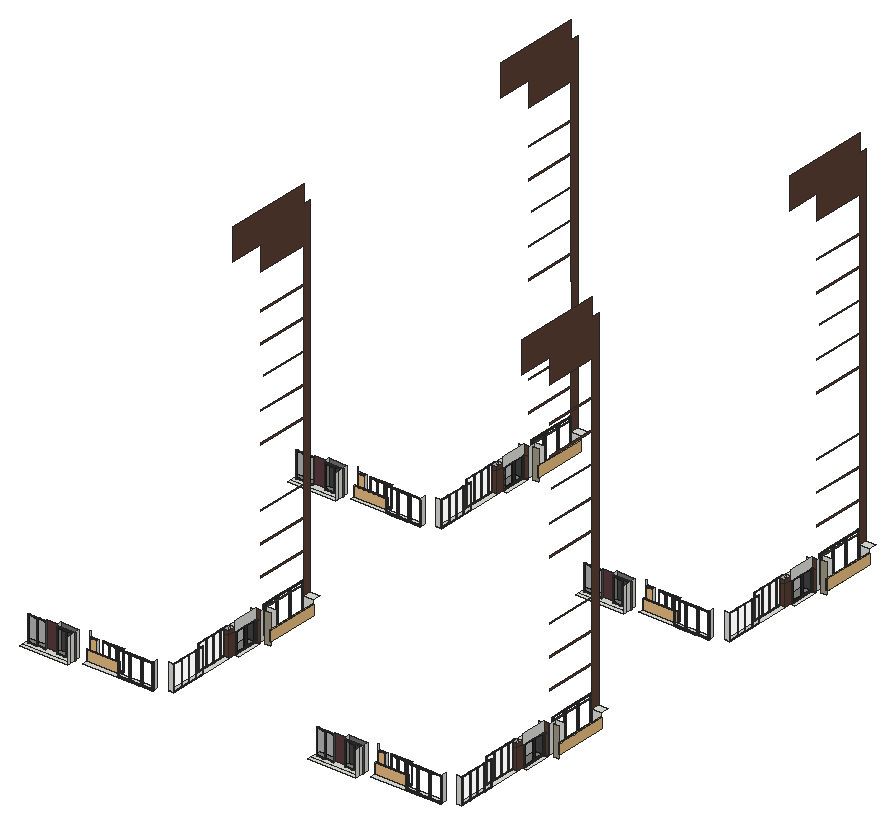
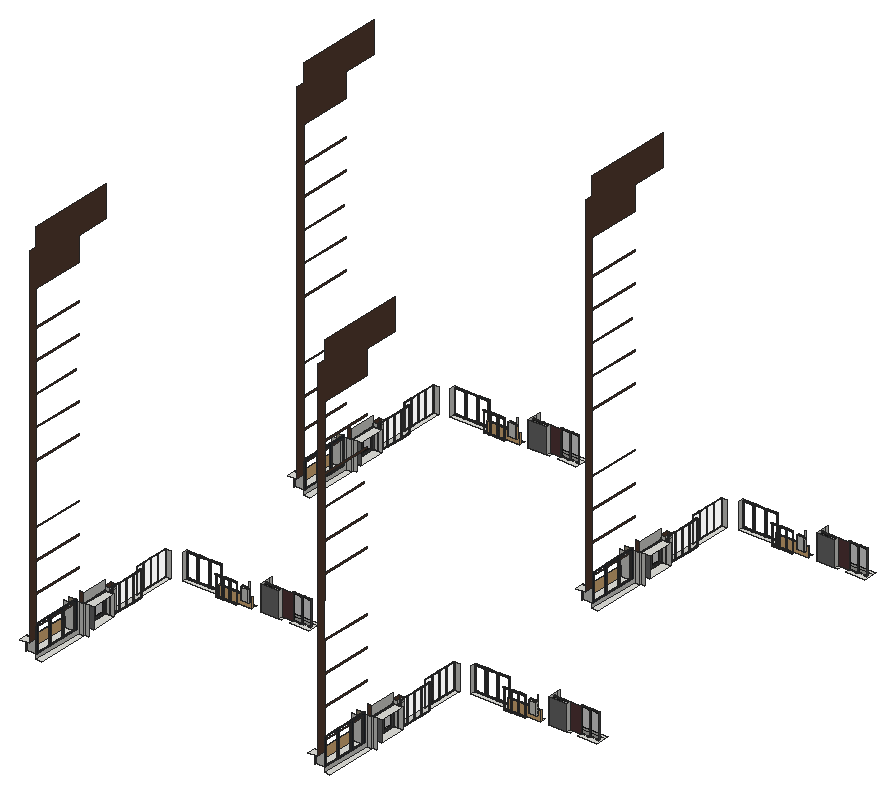
# SketchUp Ruby script. Lengths in inches.
U = 1.inch
M = Sketchup.active_model
def pt(a) = Geom::Point3d.new(a.map { |v| v * U })
def face(e, loops, mat)
  f = e.add_face(loops[0].map { |a| pt(a) })
  loops[1..].each { |l| e.add_face(l.map { |a| pt(a) }).erase! }
  f.material = f.back_material = mat if mat
  f
end
# faces: each face lists its corners as indices into pts; further lists are holes
def faces(e, pts, list, mat = nil) = list.each { |f| face(e, (f[0].is_a?(Array) ? f : [f]).map { |l| l.map { |i| pts[i] } }, mat) }
# xy, xz, yz: faces in a plane at the given z, y or x. An outline is a flat list of corners, or four numbers for a rectangle; further outlines are holes
def ring(l) = l.size == 4 ? [[l[0], l[1]], [l[2], l[1]], [l[2], l[3]], [l[0], l[3]]] : l.each_slice(2).to_a
def flat(e, list, mat, &to3) = list.each { |f| face(e, (f[0].is_a?(Array) ? f : [f]).map { |l| ring(l).map { |u, v| to3.(u, v) } }, mat) }
def xy(e, z, list, mat = nil) = flat(e, list, mat) { |x, y| [x, y, z] }
def xz(e, y, list, mat = nil) = flat(e, list, mat) { |x, z| [x, y, z] }
def yz(e, x, list, mat = nil) = flat(e, list, mat) { |y, z| [x, y, z] }
def lines(e, pts, list) = list.each { |a, b| e.add_line(pt(pts[a]), pt(pts[b])) }
# prism: a flat outline (further loops are holes) pulled along v
def prism(e, loops, v, mat = nil)
  f = face(e, loops, mat); d = Geom::Vector3d.new(v.map { |x| x * U })
  f.pushpull(f.normal.samedirection?(d) ? d.length : -d.length)
end
def box(e, o, s, mat = nil) = prism(e, [[o, [o[0] + s[0], o[1], o[2]], [o[0] + s[0], o[1] + s[1], o[2]], [o[0], o[1] + s[1], o[2]]]], [0, 0, s[2]], mat)
def at(x, y, z, deg = 0) = Geom::Transformation.translation(pt([x, y, z])) * Geom::Transformation.rotation(ORIGIN, Z_AXIS, deg.degrees)
def axes(o, x, y, z) = Geom::Transformation.new([*x, 0, *y, 0, *z, 0, *pt(o).to_a, 1])
def part(name) = M.definitions.add(name)
# library, detail: a bought-in or finely detailed component or shape, given as its bounding box
def library(name, o, s) = part(name).tap { |d| box(d.entities, o, s) }
def detail(e, o, s) = box(e.add_group.entities, o, s)
def put(e, d, t, mat = nil) = e.add_instance(d, t).tap { |i| i.material = mat if mat }
def group(e, t, mat = nil) = e.add_group.tap { |g| g.transformation = t; g.material = mat if mat }.entities
root = M.entities
M.materials.add("Glass_Tinted_Gray").color = [0, 0, 0]
M.materials["Glass_Tinted_Gray"].alpha = 0.125
M.materials.add("Glazing").color = [128, 128, 128]
M.materials["Glazing"].alpha = 0.05
M.materials.add("Powdercoating").color = [41, 44, 40]
M.materials.add("Wine2").color = [0, 0, 0]
M.materials["Wine2"].alpha = 0
M.materials.add("[0130_Gainsboro]").color = [39, 45, 50]
M.materials.add("[0135_DarkGray]").color = [81, 81, 81]
M.materials.add("[Color M05]").color = [114, 114, 114]
M.materials.add("[Concrete Tile]").color = [165, 155, 133]
M.materials.add("[Granite Brown]").color = [89, 59, 61]
M.materials.add("[Granite Brown]1").color = [89, 63, 50]
M.materials.add("[Mirror 02]").color = [229, 229, 229]
M.materials.add("[Terrazzo Light Blue]").color = [196, 214, 227]
c1 = part("PENTEK_RP Fineline 50S_Sliding_DoorCase_E1")
box(c1.entities,[0,0,0],[1.51,3.66,99.27],"[0135_DarkGray]")
c2 = part("PENTEK_RP Fineline 50S_SlidingDooe_Case_E2")
box(c2.entities,[0,0,0],[96.25,3.66,1.51],"[0135_DarkGray]")
c3 = part("pentek_RP Fineline 50S_SlidingDoor_Case")
put(c3.entities,c1,at(97.76,0,0))
put(c3.entities,c2,at(1.51,0,0))
put(c3.entities,c1,at(0,0,0))
put(c3.entities,c2,at(1.51,0,97.76))
c4 = part("PENTEK_RP Fineline 50S_SlidingDoor_GlazingBead_2")
box(c4.entities,[0,0,0],[0.56,0.59,94.39],"[0135_DarkGray]")
c5 = part("PENTEK_RP Fineline 50S_SlidingDoor_Glass")
box(c5.entities,[0,0,0],[46.58,0.16,94.39],"Glass_Tinted_Gray")
c6 = part("PENTEK_RP Fineline 50S_SlidingDoor_GlazingBead")
box(c6.entities,[0,0,0],[45.47,0.59,0.56],"[0135_DarkGray]")
c7 = part("PENTEK_RP Fineline 50S_SlidingDoor_Leaf_E1")
xy(c7.entities,0,[[0,0,0.93,1.97],[0.93,1.57,1.49,1.97]],"[0135_DarkGray]")
xy(c7.entities,96.25,[[0,0,0.93,0,0.93,1.57,1.49,1.57,1.49,1.97,0,1.97]],"[0135_DarkGray]")
xz(c7.entities,0,[[0,0,0.93,96.25]],"[0135_DarkGray]")
xz(c7.entities,1.57,[[0.93,0,1.49,95.32],[0.93,95.32,1.49,96.25]],"[0135_DarkGray]")
xz(c7.entities,1.97,[[0,0,1.49,96.25]],"[0135_DarkGray]")
yz(c7.entities,0,[[0,0,1.97,96.25]],"[0135_DarkGray]")
yz(c7.entities,0.93,[[0,0,1.57,0.93],[0,0.93,1.57,95.32],[0,95.32,1.57,96.25]],"[0135_DarkGray]")
yz(c7.entities,1.49,[[1.57,0,1.97,95.32],[1.57,95.32,1.97,96.25]],"[0135_DarkGray]")
c8 = part("PENTEK_RP Fineline 50S_SlidingDoor_Leaf_E2")
xy(c8.entities,0,[[0,0,0,1.57,0.56,1.57,0.56,1.97,46.02,1.97,46.02,1.57,46.58,1.57,46.58,0]],"[0135_DarkGray]")
xy(c8.entities,0.93,[[0,0,46.58,1.57]],"[0135_DarkGray]")
xy(c8.entities,1.49,[[0.56,1.57,46.02,1.97]],"[0135_DarkGray]")
xz(c8.entities,0,[[0,0,46.58,0.93]],"[0135_DarkGray]")
xz(c8.entities,1.57,[[0,0,0.56,0.93],[46.02,0,46.58,0.93],[0.56,0.93,46.02,1.49]],"[0135_DarkGray]")
xz(c8.entities,1.97,[[0.56,0,46.02,1.49]],"[0135_DarkGray]")
yz(c8.entities,0,[[0,0,1.57,0.93]],"[0135_DarkGray]")
yz(c8.entities,0.56,[[1.57,0,1.97,0.93],[1.57,0.93,1.97,1.49]],"[0135_DarkGray]")
yz(c8.entities,46.02,[[1.57,0,1.97,0.93],[1.57,0.93,1.97,1.49]],"[0135_DarkGray]")
yz(c8.entities,46.58,[[0,0,1.57,0.93]],"[0135_DarkGray]")
c9 = part("PENTEK_RP Fineline S_SlidingDoor_Leaf1")
put(c9.entities,c4,at(0.93,0,0.93))
put(c9.entities,c4,at(46.96,0,0.93))
put(c9.entities,c5,at(1.49,1.42,0.93))
put(c9.entities,c6,at(1.49,0,0.93))
put(c9.entities,c5,at(1.49,0.59,0.93),"[Terrazzo Light Blue]")
put(c9.entities,c7,at(0,0,0))
put(c9.entities,c7,axes([48.44,0,0],[-1,0,0],[0,1,0],[0,0,1]))
put(c9.entities,c8,axes([0.93,0,96.25],[1,0,0],[0,1,0],[0,0,-1]))
put(c9.entities,c8,at(0.93,0,0))
put(c9.entities,c6,at(1.49,0,94.77))
c10 = part("PENTEK_RP Fineline 50S_SlidingDoor_Leaf2")
put(c10.entities,c5,at(1.49,1.42,0.93))
put(c10.entities,c6,at(1.49,0,94.77))
put(c10.entities,c4,at(46.96,0,0.93))
put(c10.entities,c5,at(1.49,0.59,0.93),"[Mirror 02]")
put(c10.entities,c4,at(0.93,0,0.93))
put(c10.entities,c7,at(0,0,0))
put(c10.entities,c7,axes([48.44,0,0],[-1,0,0],[0,1,0],[0,0,1]))
put(c10.entities,c6,at(1.49,0,0.93))
put(c10.entities,c8,axes([0.93,0,96.25],[1,0,0],[0,1,0],[0,0,-1]))
put(c10.entities,c8,at(0.93,0,0))
c11 = part("PENTEK - Slimmest Steel Sliding Door / Window\#1")
put(c11.entities,c3,at(0,-1.88,-0.09))
put(c11.entities,c9,at(1.51,-2.27,1.42))
put(c11.entities,c10,at(49.32,-0.3,1.42))
c12 = part("Group\#15")
xy(c12.entities,0,[[0,-55.94,0.71,45.94]])
xy(c12.entities,0.2,[[0,-55.94,0.47,45.94],[0.47,45.94,0.71,46.42]])
xy(c12.entities,2.36,[[0.47,-55.94,0.71,46.42]])
xz(c12.entities,-55.94,[[0,0,0.71,0,0.71,2.36,0.47,2.36,0.47,0.2,0,0.2]])
xz(c12.entities,45.94,[[0,0,0.71,0.2]])
xz(c12.entities,46.42,[[0.47,0.2,0.71,2.36]])
yz(c12.entities,0,[[-55.94,0,45.94,0.2]])
yz(c12.entities,0.47,[[-55.94,0.2,46.42,2.36]])
yz(c12.entities,0.71,[[-55.94,0,45.94,0,45.94,0.2,46.42,0.2,46.42,2.36,-55.94,2.36]])
c13 = part("Group\#7")
xy(c13.entities,0,[[0,-59.09,0.71,45.94]])
xy(c13.entities,0.2,[[0,-59.09,0.47,45.94],[0.47,45.94,0.71,46.42]])
xy(c13.entities,2.36,[[0.47,-59.09,0.71,46.42]])
xz(c13.entities,-59.09,[[0,0,0.71,0,0.71,2.36,0.47,2.36,0.47,0.2,0,0.2]])
xz(c13.entities,45.94,[[0,0,0.71,0.2]])
xz(c13.entities,46.42,[[0.47,0.2,0.71,2.36]])
yz(c13.entities,0,[[-59.09,0,45.94,0.2]])
yz(c13.entities,0.47,[[-59.09,0.2,46.42,2.36]])
yz(c13.entities,0.71,[[-59.09,0,45.94,0,45.94,0.2,46.42,0.2,46.42,2.36,-59.09,2.36]])
c14 = part("Group\#16")
prism(c14.entities,[[[0.47,-56.18,0.2],[0,-56.18,0.2],[0,-56.18,0],[0.71,-56.18,0],[0.71,-56.18,2.36],[0.47,-56.18,2.36]]],[0,28.68,0])
c15 = part("Group\#10")
box(c15.entities,[-0.73,0,0],[27.99,0.55,102.05])
c16 = part("Group\#18")
xy(c16.entities,0,[[0.47,-56.18,0.47,-55.47,0,-55.47,0,-28.21,1.18,-28.21,1.18,-56.18]])
xy(c16.entities,0.2,[[0.71,-56.18,1.18,-28.21],[0,-55.47,0.47,-28.21],[0.47,-28.21,0.71,-27.74]])
xy(c16.entities,2.36,[[0.47,-56.18,0.71,-27.74]])
xz(c16.entities,-56.18,[[0.47,0,1.18,0,1.18,0.2,0.71,0.2,0.71,2.36,0.47,2.36]])
xz(c16.entities,-55.47,[[0,0,0.47,0.2]])
xz(c16.entities,-28.21,[[0,0,1.18,0.2]])
xz(c16.entities,-27.74,[[0.47,0.2,0.71,2.36]])
yz(c16.entities,0,[[-55.47,0,-28.21,0.2]])
yz(c16.entities,0.47,[[-56.18,0,-55.47,0.2],[-56.18,0.2,-27.74,2.36]])
yz(c16.entities,0.71,[[-56.18,0.2,-27.74,2.36]])
yz(c16.entities,1.18,[[-56.18,0,-28.21,0.2]])
c17 = part("Group\#34")
xy(c17.entities,0,[[-20.45,0,7.76,1.22]])
xy(c17.entities,0.06,[[-20.39,0.06,7.7,1.22]])
xy(c17.entities,0.47,[[-19.98,0,7.28,0.06]])
xy(c17.entities,101.89,[[-19.98,0,7.28,0.06]])
xy(c17.entities,102.3,[[-20.39,0.06,7.7,1.22]])
xy(c17.entities,102.36,[[-20.45,0,7.76,1.22]])
xz(c17.entities,0,[[[-20.45,0,7.76,102.36],[-19.98,0.47,7.28,101.89]]])
xz(c17.entities,0.06,[[[-20.39,0.06,7.7,102.3],[-19.98,0.47,7.28,101.89]]])
xz(c17.entities,1.22,[[[-20.45,0,7.76,102.36],[-20.39,0.06,7.7,102.3]]])
yz(c17.entities,-20.45,[[0,0,1.22,102.36]])
yz(c17.entities,-20.39,[[0.06,0.06,1.22,102.3]])
yz(c17.entities,-19.98,[[0,0.47,0.06,101.89]])
yz(c17.entities,7.28,[[0,0.47,0.06,101.89]])
yz(c17.entities,7.7,[[0.06,0.06,1.22,102.3]])
yz(c17.entities,7.76,[[0,0,1.22,102.36]])
c18 = part("Group\#6")
put(c18.entities,c12,axes([27.97,0,7.875],[1,0,0],[0,0,-1],[0,1,0]),"Powdercoating")
put(c18.entities,c13,axes([0.71,0,6.8],[-1,0,0],[0,0,-0.97687],[0,1,0]),"Powdercoating")
put(c18.entities,c14,axes([-27.5,0,-38.07],[0,0,-1],[-1,0,0],[0,1,0]),"Powdercoating")
put(c18.entities,c15,at(1.12,0.35,-38.39),"Glazing")
put(c18.entities,c16,axes([-27.5,0,63.35],[0,0,1],[-1,0,0],[0,1,0]),"Powdercoating")
put(c18.entities,c17,at(20.6875,1.0625,-38.54),"Powdercoating")
c19 = part("Sliding door assembly")
put(c19.entities,c18,at(-1.18,4.5,38.86))
g1 = group(c19.entities,at(84.74,4.5,38.86))
put(g1,c12,axes([-27.97,0,7.875],[-1,0,0],[0,0,-1],[0,1,0]),"Powdercoating")
put(g1,c13,axes([-0.71,0,6.8],[1,0,0],[0,0,-0.97687],[0,1,0]),"Powdercoating")
put(g1,c14,axes([27.5,0,-38.07],[0,0,-1],[1,0,0],[0,1,0]),"Powdercoating")
put(g1,c15,axes([-1.12,0.35,-38.39],[-1,0,0],[0,1,0],[0,0,1]),"Glazing")
put(g1,c16,axes([27.5,0,63.35],[0,0,1],[1,0,0],[0,1,0]),"Powdercoating")
put(g1,c17,axes([-20.6875,1.0625,-38.54],[-1,0,0],[0,1,0],[0,0,1]),"Powdercoating")
g2 = group(c19.entities,at(56.0625,4.5,38.86))
put(g2,c12,axes([-27.97,0,7.875],[-1,0,0],[0,0,-1],[0,1,0]),"Powdercoating")
put(g2,c14,axes([27.5,0,-38.07],[0,0,-1],[1,0,0],[0,1,0]),"Powdercoating")
put(g2,c15,axes([-1.12,0.35,-38.39],[-1,0,0],[0,1,0],[0,0,1]),"Glazing")
put(g2,c16,axes([27.5,0,63.35],[0,0,1],[1,0,0],[0,1,0]),"Powdercoating")
put(g2,c17,axes([-20.6875,1.0625,-38.54],[-1,0,0],[0,1,0],[0,0,1]),"Powdercoating")
g3 = group(g2,at(-0.71,0,6.8),"Powdercoating")
xy(g3,-45.34,[[0.47,0.2,0.71,2.36]])
xy(g3,-44.88,[[0,0,0.71,0.2]])
xy(g3,57.73,[[0,0,0.71,0,0.71,2.36,0.47,2.36,0.47,0.2,0,0.2]])
xz(g3,0,[[0,-44.88,0.71,57.73]])
xz(g3,0.2,[[0.47,-45.34,0.71,-44.88],[0,-44.88,0.47,57.73]])
xz(g3,2.36,[[0.47,-45.34,0.71,57.73]])
yz(g3,0,[[0,-44.88,0.2,57.73]])
yz(g3,0.47,[[0.2,-45.34,2.36,57.73]])
yz(g3,0.71,[[0.2,-45.34,2.36,-45.34,2.36,57.73,0,57.73,0,-44.88,0.2,-44.88]])
put(c19.entities,c18,axes([-33.94,4.5,38.86],[1.14218,0,0],[0,1,0],[0,0,1]))
c20 = part("sliding door")
put(c20.entities,c19,at(0,-4.5,-0.08))
c21 = part("Framed glazing panel")
xy(c21.entities,0,[[0,-0.98,43.07,0],[0,0,43.07,1.4]],"[0130_Gainsboro]")
xy(c21.entities,0.3,[[0.3,-1.43,42.77,-0.98]],"[0130_Gainsboro]")
xy(c21.entities,2.95,[[2.95,-1.43,40.12,-0.63],[2.95,-0.63,40.12,0],[2.95,0,40.12,0.64],[2.95,0.64,40.12,1.4]],"[0130_Gainsboro]")
xy(c21.entities,3.54,[[3.54,-0.63,39.53,0],[3.54,0,39.53,0.64]],"[0130_Gainsboro]")
xy(c21.entities,111.8125,[[3.54,-0.63,39.53,0],[3.54,0,39.53,0.64]],"[0130_Gainsboro]")
xy(c21.entities,112.4,[[2.95,-1.43,40.12,-0.63],[2.95,-0.63,40.12,0],[2.95,0,40.12,0.64],[2.95,0.64,40.12,1.4]],"[0130_Gainsboro]")
xy(c21.entities,115.05,[[0.3,-1.43,42.77,-0.98]],"[0130_Gainsboro]")
xy(c21.entities,115.35,[[0,-0.98,43.07,0],[0,0,43.07,1.4]],"[0130_Gainsboro]")
xz(c21.entities,-1.43,[[[0.3,0.3,42.77,115.05],[2.95,2.95,40.12,112.4]]],"[0130_Gainsboro]")
xz(c21.entities,-0.98,[[[0,0,43.07,115.35],[0.3,0.3,42.77,115.05]]],"[0130_Gainsboro]")
xz(c21.entities,-0.63,[[[2.95,2.95,40.12,112.4],[3.54,3.54,39.53,111.8125]]],"[0130_Gainsboro]")
xz(c21.entities,0,[[3.54,3.54,39.53,111.8125]],"Wine2")
xz(c21.entities,0,[[[0,0,43.07,115.35],[2.95,2.95,40.12,112.4]],[[2.95,2.95,40.12,112.4],[3.54,3.54,39.53,111.8125]]],"[0130_Gainsboro]")
xz(c21.entities,0.64,[[[2.95,2.95,40.12,112.4],[3.54,3.54,39.53,111.8125]]],"[0130_Gainsboro]")
xz(c21.entities,1.4,[[[0,0,43.07,115.35],[2.95,2.95,40.12,112.4]]],"[0130_Gainsboro]")
yz(c21.entities,0,[[-0.98,0,0,115.35],[0,0,1.4,115.35]],"[0130_Gainsboro]")
yz(c21.entities,0.3,[[-1.43,0.3,-0.98,115.05]],"[0130_Gainsboro]")
yz(c21.entities,2.95,[[-1.43,2.95,-0.63,112.4],[-0.63,2.95,0,112.4],[0,2.95,0.64,112.4],[0.64,2.95,1.4,112.4]],"[0130_Gainsboro]")
yz(c21.entities,3.54,[[-0.63,3.54,0,111.8125],[0,3.54,0.64,111.8125]],"[0130_Gainsboro]")
yz(c21.entities,39.53,[[-0.63,3.54,0,111.8125],[0,3.54,0.64,111.8125]],"[0130_Gainsboro]")
yz(c21.entities,40.12,[[-1.43,2.95,-0.63,112.4],[-0.63,2.95,0,112.4],[0,2.95,0.64,112.4],[0.64,2.95,1.4,112.4]],"[0130_Gainsboro]")
yz(c21.entities,42.77,[[-1.43,0.3,-0.98,115.05]],"[0130_Gainsboro]")
yz(c21.entities,43.07,[[-0.98,0,0,115.35],[0,0,1.4,115.35]],"[0130_Gainsboro]")
c22 = part("Glazed panel assembly")
put(c22.entities,c21,axes([90.57,1.43,0],[1.05148,0,0],[0,1,0],[0,0,1]))
put(c22.entities,c21,axes([0,1.43,0],[1.05148,0,0],[0,1,0],[0,0,1]))
put(c22.entities,c21,axes([45.29,1.43,0],[1.05148,0,0],[0,1,0],[0,0,1]))
c23 = library("Glass Railing",[0,0,0],[139.5,4.76,42])
c24 = library("Klein+raam",[128.36,12.7,0],[19.68,5.51,55.12])
xy(root,259.75,[[890.875,2295.875,913.875,2518.89],[2109.0625,2295.875,2132.0625,2518.89],[890.875,3710.5625,913.875,3933.57],[2109.0625,3710.5625,2132.0625,3933.57]])
xy(root,271.5,[[894.3125,1835.1875,913.875,2156.01],[2112.5,1835.1875,2132.0625,2156.01],[913.875,2156.01,930.75,2266.33],[2132.0625,2156.01,2148.9375,2266.33],[894.3125,3249.875,913.875,3570.7],
  [2112.5,3249.875,2132.0625,3570.7],[913.875,3570.7,930.75,3681.01],[2132.0625,3570.7,2148.9375,3681.01]])
xy(root,271.9375,[[320.25,1763.25,523.04,1763.25,523.04,1822.9375,445.4,1822.9375,445.4,1806.5625,399.91,1806.5625,399.91,1822.9375,320.25,1822.9375],[1538.44,1763.25,1741.23,1763.25,1741.23,1822.9375,1663.58,1822.9375,1663.58,1806.5625,1618.1,1806.5625,1618.1,1822.9375,1538.44,1822.9375],[431.33,1806.5625,445.4,1822.9375],[1649.52,1806.5625,1663.58,1822.9375],[320.25,3177.9375,523.04,3177.9375,523.04,3237.625,445.4,3237.625,445.4,3221.25,399.91,3221.25,399.91,3237.625,320.25,3237.625],
  [1538.44,3177.9375,1741.23,3177.9375,1741.23,3237.625,1663.58,3237.625,1663.58,3221.25,1618.1,3221.25,1618.1,3237.625,1538.44,3237.625],[431.33,3221.25,445.4,3237.625],[1649.52,3221.25,1663.58,3237.625]])
xy(root,272.125,[[557.88,1799.9375,852.75,1822.9375],[1776.07,1799.9375,2070.9375,1822.9375],[557.88,3214.625,852.75,3237.625],[1776.07,3214.625,2070.9375,3237.625]])
xy(root,275.36,[[874.375,2156.01,913.875,2266.33],[2092.5625,2156.01,2132.0625,2266.33],[874.375,3570.7,913.875,3681.01],[2092.5625,3570.7,2132.0625,3681.01]])
xy(root,280.3125,[[913.875,2321.98,954.6875,2518.89],[2132.0625,2321.98,2172.875,2518.89],[913.875,3736.67,954.6875,3933.57],[2132.0625,3736.67,2172.875,3933.57]])
xy(root,301.74,[[557.4,1835.1875,589.71,1845.8125],[1775.59,1835.1875,1807.9,1845.8125],[557.4,3249.875,589.71,3260.5],[1775.59,3249.875,1807.9,3260.5]])
xy(root,336.0625,[[913.875,2518.89,954.6875,2554.375],[2132.0625,2518.89,2172.875,2554.375],[913.875,3933.57,954.6875,3969.0625],[2132.0625,3933.57,2172.875,3969.0625]])
xy(root,354.03,[[557.4,1835.1875,589.71,1845.8125],[1775.59,1835.1875,1807.9,1845.8125],[557.4,3249.875,589.71,3260.5],[1775.59,3249.875,1807.9,3260.5]])
xy(root,358.625,[[611.65,1835.1875,701.59,1839.6875],[1829.84,1835.1875,1919.77,1839.6875],[611.65,3249.875,701.59,3254.375],[1829.84,3249.875,1919.77,3254.375]])
xy(root,361.04,[[894.3125,2124.51,913.875,2156.01],[2112.5,2124.51,2132.0625,2156.01],[874.375,2156.01,913.875,2266.33],[2092.5625,2156.01,2132.0625,2266.33],[894.3125,3539.2,913.875,3570.7],
  [2112.5,3539.2,2132.0625,3570.7],[874.375,3570.7,913.875,3681.01],[2092.5625,3570.7,2132.0625,3681.01]])
xz(root,1806.5625,[[399.98,271.9375,445.4,271.9375,445.4,378,400.51,378],[1618.17,271.9375,1663.58,271.9375,1663.58,378,1618.7,378]],"[Granite Brown]")
xz(root,1822.9375,[[445.4,271.9375,523.04,378],[1663.58,271.9375,1741.23,378]],"[Color M05]")
xz(root,1835.1875,[[890.875,271.5,913.875,378],[2109.0625,271.5,2132.0625,378]])
xz(root,1835.1875,[[557.4,301.74,557.88,354.03],[1775.59,301.74,1776.07,354.03],[557.4,354.03,557.88,377],[1775.59,354.03,1776.07,377]],"[Granite Brown]")
xz(root,1845.8125,[[557.4,301.74,589.71,354.03],[1775.59,301.74,1807.9,354.03]])
xz(root,2124.51,[[894.3125,275.36,913.875,361.04],[2112.5,275.36,2132.0625,361.04],[894.3125,361.04,913.875,378],[2112.5,361.04,2132.0625,378]],"[Granite Brown]1")
xz(root,2156.01,[[894.3125,271.5,913.875,275.36],[2112.5,271.5,2132.0625,275.36],[874.375,275.36,894.3125,361.04],[894.3125,275.36,913.875,361.04],[2092.5625,275.36,2112.5,361.04],
  [2112.5,275.36,2132.0625,361.04],[894.3125,361.04,913.875,378],[2112.5,361.04,2132.0625,378]])
xz(root,2266.33,[[913.875,271.5,930.75,275.36],[2132.0625,271.5,2148.9375,275.36]])
xz(root,2266.33,[[874.375,275.36,913.875,361.04],[2092.5625,275.36,2132.0625,361.04]],"[Color M05]")
xz(root,2266.33,[[913.875,275.36,930.75,361.04],[2132.0625,275.36,2148.9375,361.04],[913.875,361.04,930.75,401.36],[2132.0625,361.04,2148.9375,401.36]],"[Granite Brown]1")
xz(root,2290,[[874.375,259.75,890.875,378],[2092.5625,259.75,2109.0625,378]])
xz(root,2295.875,[[890.875,259.75,913.875,378],[2109.0625,259.75,2132.0625,378]])
xz(root,2295.875,[[930.75,259.75,954.6875,384],[2148.9375,259.75,2172.875,384]],"[Concrete Tile]")
xz(root,2321.98,[[913.875,280.3125,954.6875,384],[2132.0625,280.3125,2172.875,384]])
xz(root,2518.89,[[913.875,280.3125,954.6875,336.0625],[2132.0625,280.3125,2172.875,336.0625]])
xz(root,3221.25,[[399.98,271.9375,445.4,271.9375,445.4,378,400.51,378],[1618.17,271.9375,1663.58,271.9375,1663.58,378,1618.7,378]],"[Granite Brown]")
xz(root,3237.625,[[445.4,271.9375,523.04,378],[1663.58,271.9375,1741.23,378]],"[Color M05]")
xz(root,3249.875,[[890.875,271.5,913.875,378],[2109.0625,271.5,2132.0625,378]])
xz(root,3249.875,[[557.4,301.74,557.88,354.03],[1775.59,301.74,1776.07,354.03],[557.4,354.03,557.88,377],[1775.59,354.03,1776.07,377]],"[Granite Brown]")
xz(root,3260.5,[[557.4,301.74,589.71,354.03],[1775.59,301.74,1807.9,354.03]])
xz(root,3539.2,[[894.3125,275.36,913.875,361.04],[2112.5,275.36,2132.0625,361.04],[894.3125,361.04,913.875,378],[2112.5,361.04,2132.0625,378]],"[Granite Brown]1")
xz(root,3570.7,[[894.3125,271.5,913.875,275.36],[2112.5,271.5,2132.0625,275.36],[874.375,275.36,894.3125,361.04],[894.3125,275.36,913.875,361.04],[2092.5625,275.36,2112.5,361.04],
  [2112.5,275.36,2132.0625,361.04],[894.3125,361.04,913.875,378],[2112.5,361.04,2132.0625,378]])
xz(root,3681.01,[[913.875,271.5,930.75,275.36],[2132.0625,271.5,2148.9375,275.36]])
xz(root,3681.01,[[874.375,275.36,913.875,361.04],[2092.5625,275.36,2132.0625,361.04]],"[Color M05]")
xz(root,3681.01,[[913.875,275.36,930.75,361.04],[2132.0625,275.36,2148.9375,361.04],[913.875,361.04,930.75,401.36],[2132.0625,361.04,2148.9375,401.36]],"[Granite Brown]1")
xz(root,3704.6875,[[874.375,259.75,890.875,378],[2092.5625,259.75,2109.0625,378]])
xz(root,3710.5625,[[890.875,259.75,913.875,378],[2109.0625,259.75,2132.0625,378]])
xz(root,3710.5625,[[930.75,259.75,954.6875,384],[2148.9375,259.75,2172.875,384]],"[Concrete Tile]")
xz(root,3736.67,[[913.875,280.3125,954.6875,384],[2132.0625,280.3125,2172.875,384]])
xz(root,3933.57,[[913.875,280.3125,954.6875,336.0625],[2132.0625,280.3125,2172.875,336.0625]])
yz(root,445.4,[[1806.5625,271.9375,1822.9375,378],[3221.25,271.9375,3237.625,378]])
yz(root,523.04,[[1763.25,271.9375,1822.9375,378],[3177.9375,271.9375,3237.625,378]])
yz(root,557.4,[[1835.1875,301.74,1839.6875,354.03],[1839.6875,301.74,1845.8125,354.03],[3249.875,301.74,3254.375,354.03],[3254.375,301.74,3260.5,354.03],[1835.1875,354.03,1839.6875,378],
  [3249.875,354.03,3254.375,378]])
yz(root,589.71,[[1835.1875,301.74,1845.8125,354.03],[3249.875,301.74,3260.5,354.03]])
yz(root,852.75,[[1799.9375,272.125,1822.9375,378],[3214.625,272.125,3237.625,378]])
yz(root,890.875,[[2290,259.75,2295.875,378],[3704.6875,259.75,3710.5625,378]])
yz(root,894.3125,[[2124.51,271.5,2148.83,275.36],[2148.83,271.5,2156.01,275.36],[3539.2,271.5,3563.51,275.36],[3563.51,271.5,3570.7,275.36],[2124.51,275.36,2148.83,361.04],
  [2148.83,275.36,2156.01,361.04],[3539.2,275.36,3563.51,361.04],[3563.51,275.36,3570.7,361.04],[2124.51,361.04,2148.83,378],[2148.83,361.04,2156.01,378],
  [3539.2,361.04,3563.51,378],[3563.51,361.04,3570.7,378]])
yz(root,913.875,[[2295.875,259.75,2295.875,378,2321.98,378,2321.98,280.3125,2518.89,280.3125,2518.89,259.75],[3710.5625,259.75,3710.5625,378,3736.67,378,3736.67,280.3125,3933.57,280.3125,3933.57,259.75],[2156.01,271.5,2266.33,275.36],[3570.7,271.5,3681.01,275.36],[2156.01,361.04,2266.33,401.36],
  [3570.7,361.04,3681.01,401.36]])
yz(root,913.875,[[2124.51,271.5,2156.01,361.04],[3539.2,271.5,3570.7,361.04],[2518.89,336.0625,2554.375,336.0625,2554.375,1821.625,2518.89,1821.625,2518.89,1895.25,2148.83,1895.25,2148.83,1764,2295.875,1764,2295.875,1663.0625,2518.89,1663.0625,2518.89,1518,2295.875,1518,2295.875,1512,2518.89,1512,2518.89,1392,2295.875,1392,2295.875,1386,2518.89,1386,2518.89,1266,2310.68,1266,2310.68,1260,2518.89,1260,2518.89,1140,2295.875,1140,2295.875,1134,2518.89,1134,2518.89,1014,2295.875,1014,2295.875,1008,2519.125,1008,2519.125,908.8125,2520.14,908.8125,2520.14,762,2295.875,762,2295.875,756,2518.89,756,2518.89,636,2295.875,636,2295.875,630,2518.89,630,2518.89,510,2295.875,510,2295.875,504,2518.89,504,2518.89,384,2321.98,384,2321.98,378,2518.89,378],[3933.57,336.0625,3969.0625,336.0625,3969.0625,1821.625,3933.57,1821.625,3933.57,1895.25,3563.51,1895.25,3563.51,1764,3710.5625,1764,3710.5625,1663.0625,3933.57,1663.0625,3933.57,1518,3710.5625,1518,3710.5625,1512,3933.57,1512,3933.57,1392,3710.5625,1392,3710.5625,1386,3933.57,1386,3933.57,1266,3725.37,1266,3725.37,1260,3933.57,1260,3933.57,1140,3710.5625,1140,3710.5625,1134,3933.57,1134,3933.57,1014,3710.5625,1014,3710.5625,1008,3933.8125,1008,3933.8125,908.8125,3934.82,908.8125,3934.82,762,3710.5625,762,3710.5625,756,3933.57,756,3933.57,636,3710.5625,636,3710.5625,630,3933.57,630,3933.57,510,3710.5625,510,3710.5625,504,3933.57,504,3933.57,384,3736.67,384,3736.67,378,3933.57,378],[2124.51,361.04,2156.01,378],
  [3539.2,361.04,3570.7,378]],"[Granite Brown]1")
yz(root,1663.58,[[1806.5625,271.9375,1822.9375,378],[3221.25,271.9375,3237.625,378]])
yz(root,1741.23,[[1763.25,271.9375,1822.9375,378],[3177.9375,271.9375,3237.625,378]])
yz(root,1775.59,[[1835.1875,301.74,1839.6875,354.03],[1839.6875,301.74,1845.8125,354.03],[3249.875,301.74,3254.375,354.03],[3254.375,301.74,3260.5,354.03],[1835.1875,354.03,1839.6875,378],
  [3249.875,354.03,3254.375,378]])
yz(root,1807.9,[[1835.1875,301.74,1845.8125,354.03],[3249.875,301.74,3260.5,354.03]])
yz(root,2070.9375,[[1799.9375,272.125,1822.9375,378],[3214.625,272.125,3237.625,378]])
yz(root,2109.0625,[[2290,259.75,2295.875,378],[3704.6875,259.75,3710.5625,378]])
yz(root,2112.5,[[2124.51,271.5,2148.83,275.36],[2148.83,271.5,2156.01,275.36],[3539.2,271.5,3563.51,275.36],[3563.51,271.5,3570.7,275.36],[2124.51,275.36,2148.83,361.04],
  [2148.83,275.36,2156.01,361.04],[3539.2,275.36,3563.51,361.04],[3563.51,275.36,3570.7,361.04],[2124.51,361.04,2148.83,378],[2148.83,361.04,2156.01,378],
  [3539.2,361.04,3563.51,378],[3563.51,361.04,3570.7,378]])
yz(root,2132.0625,[[2295.875,259.75,2295.875,378,2321.98,378,2321.98,280.3125,2518.89,280.3125,2518.89,259.75],[3710.5625,259.75,3710.5625,378,3736.67,378,3736.67,280.3125,3933.57,280.3125,3933.57,259.75],[2156.01,271.5,2266.33,275.36],[3570.7,271.5,3681.01,275.36],[2156.01,361.04,2266.33,401.36],
  [3570.7,361.04,3681.01,401.36]])
yz(root,2132.0625,[[2124.51,271.5,2156.01,361.04],[3539.2,271.5,3570.7,361.04],[2518.89,336.0625,2554.375,336.0625,2554.375,1821.625,2518.89,1821.625,2518.89,1895.25,2148.83,1895.25,2148.83,1764,2295.875,1764,2295.875,1663.0625,2518.89,1663.0625,2518.89,1518,2295.875,1518,2295.875,1512,2518.89,1512,2518.89,1392,2295.875,1392,2295.875,1386,2518.89,1386,2518.89,1266,2310.68,1266,2310.68,1260,2518.89,1260,2518.89,1140,2295.875,1140,2295.875,1134,2518.89,1134,2518.89,1014,2295.875,1014,2295.875,1008,2519.125,1008,2519.125,908.8125,2520.14,908.8125,2520.14,762,2295.875,762,2295.875,756,2518.89,756,2518.89,636,2295.875,636,2295.875,630,2518.89,630,2518.89,510,2295.875,510,2295.875,504,2518.89,504,2518.89,384,2321.98,384,2321.98,378,2518.89,378],[3933.57,336.0625,3969.0625,336.0625,3969.0625,1821.625,3933.57,1821.625,3933.57,1895.25,3563.51,1895.25,3563.51,1764,3710.5625,1764,3710.5625,1663.0625,3933.57,1663.0625,3933.57,1518,3710.5625,1518,3710.5625,1512,3933.57,1512,3933.57,1392,3710.5625,1392,3710.5625,1386,3933.57,1386,3933.57,1266,3725.37,1266,3725.37,1260,3933.57,1260,3933.57,1140,3710.5625,1140,3710.5625,1134,3933.57,1134,3933.57,1014,3710.5625,1014,3710.5625,1008,3933.8125,1008,3933.8125,908.8125,3934.82,908.8125,3934.82,762,3710.5625,762,3710.5625,756,3933.57,756,3933.57,636,3710.5625,636,3710.5625,630,3933.57,630,3933.57,510,3710.5625,510,3710.5625,504,3933.57,504,3933.57,384,3736.67,384,3736.67,378,3933.57,378],[2124.51,361.04,2156.01,378],
  [3539.2,361.04,3570.7,378]],"[Granite Brown]1")
p = [[1741.23,1778.3125,271.9375],[1741.23,1778.3125,378],[1538.44,1778.3125,271.9375],[523.04,1778.3125,271.9375],[523.04,1778.3125,378],[320.25,1778.3125,271.9375],
  [1741.23,3193,271.9375],[1741.23,3193,378],[1538.44,3193,271.9375],[523.04,3193,271.9375],[523.04,3193,378],[320.25,3193,271.9375]]
lines(root,p,[[0,1],[2,0],[3,4],[5,3],[6,7],[8,6],[9,10],[11,9]])
put(root,c11,axes([1545.45,1800.2,268.88],[0.75346,0,0],[0,0.88,0],[0,0,1.1067]))
put(root,c11,axes([327.26,1800.2,268.88],[0.75346,0,0],[0,0.88,0],[0,0,1.1067]))
put(root,c11,axes([1545.45,3214.89,268.88],[0.75346,0,0],[0,0.88,0],[0,0,1.1067]))
put(root,c11,axes([327.26,3214.89,268.88],[0.75346,0,0],[0,0.88,0],[0,0,1.1067]))
put(root,c11,axes([1666.41,1800.2,269.46],[0.77709,0,0],[0,0.88,0],[0,0,1.054]))
put(root,c11,axes([448.22,1800.2,269.46],[0.77709,0,0],[0,0.88,0],[0,0,1.054]))
put(root,c11,axes([1666.41,3214.89,269.46],[0.77709,0,0],[0,0.88,0],[0,0,1.054]))
put(root,c11,axes([448.22,3214.89,269.46],[0.77709,0,0],[0,0.88,0],[0,0,1.054]))
put(root,c20,axes([2109.0625,2037.39,270.78],[0,1.302,0],[-1,0,0],[0,0,1.03877]))
put(root,c20,axes([890.875,2037.39,270.78],[0,1.302,0],[-1,0,0],[0,0,1.03877]))
put(root,c20,axes([2109.0625,3452.08,270.78],[0,1.302,0],[-1,0,0],[0,0,1.03877]))
put(root,c20,axes([890.875,3452.08,270.78],[0,1.302,0],[-1,0,0],[0,0,1.03877]))
put(root,c20,axes([2132.0625,1879.38,271.5],[0,1.302,0],[-1,0,0],[0,0,1.03877]))
put(root,c20,axes([913.875,1879.38,271.5],[0,1.302,0],[-1,0,0],[0,0,1.03877]))
put(root,c20,axes([2132.0625,3294.06,271.5],[0,1.302,0],[-1,0,0],[0,0,1.03877]))
put(root,c20,axes([913.875,3294.06,271.5],[0,1.302,0],[-1,0,0],[0,0,1.03877]))
put(root,c22,axes([1829.4375,1835.1875,272.125],[0.6649,0,0],[0,0.61,0],[0,0,0.74986]))
put(root,c22,axes([611.25,1835.1875,272.125],[0.6649,0,0],[0,0.61,0],[0,0,0.74986]))
put(root,c22,axes([1829.4375,3249.875,272.125],[0.6649,0,0],[0,0.61,0],[0,0,0.74986]))
put(root,c22,axes([611.25,3249.875,272.125],[0.6649,0,0],[0,0.61,0],[0,0,0.74986]))
put(root,c22,axes([1923.26,1799.9375,272.125],[1.09,0,0],[0,1,0],[0,0,0.91782]))
put(root,c23,at(1774.12,1820.19,272.125))
put(root,c22,axes([705.08,1799.9375,272.125],[1.09,0,0],[0,1,0],[0,0,0.91782]))
put(root,c23,at(555.93,1820.19,272.125))
put(root,c23,at(1774.12,3234.88,272.125))
put(root,c22,axes([1923.26,3214.625,272.125],[1.09,0,0],[0,1,0],[0,0,0.91782]))
put(root,c22,axes([705.08,3214.625,272.125],[1.09,0,0],[0,1,0],[0,0,0.91782]))
put(root,c23,at(555.93,3234.88,272.125))
put(root,c11,axes([2131.3,2157.7,274.11],[0,1.12181,0],[-2.51374,0,0],[0,0,0.87918]),"[Granite Brown]1")
put(root,c11,axes([913.11,2157.7,274.11],[0,1.12181,0],[-2.51374,0,0],[0,0,0.87918]),"[Granite Brown]1")
put(root,c11,axes([2131.3,3572.39,274.11],[0,1.12181,0],[-2.51374,0,0],[0,0,0.87918]),"[Granite Brown]1")
put(root,c11,axes([913.11,3572.39,274.11],[0,1.12181,0],[-2.51374,0,0],[0,0,0.87918]),"[Granite Brown]1")
put(root,c23,axes([2174.88,2295.6875,277.43],[0,1.6,0],[-1,0,0],[0,0,1]))
put(root,c23,axes([956.7,2295.6875,277.43],[0,1.6,0],[-1,0,0],[0,0,1]))
put(root,c23,axes([2174.88,3710.375,277.43],[0,1.6,0],[-1,0,0],[0,0,1]))
put(root,c23,axes([956.7,3710.375,277.43],[0,1.6,0],[-1,0,0],[0,0,1]))
put(root,c22,axes([2132.0625,2309.55,280.3125],[0,1.54079,0],[-1,0,0],[0,0,1]))
put(root,c22,axes([913.875,2309.55,280.3125],[0,1.54079,0],[-1,0,0],[0,0,1]))
put(root,c22,axes([2132.0625,3724.24,280.3125],[0,1.54079,0],[-1,0,0],[0,0,1]))
put(root,c22,axes([913.875,3724.24,280.3125],[0,1.54079,0],[-1,0,0],[0,0,1]))
put(root,c24,axes([1571.78,1826.29,299.35],[1.58777,0,0],[0,0.68,0],[0,0,0.99202]))
put(root,c24,axes([353.6,1826.29,299.35],[1.58777,0,0],[0,0.68,0],[0,0,0.99202]))
put(root,c24,axes([1571.78,3240.97,299.35],[1.58777,0,0],[0,0.68,0],[0,0,0.99202]))
put(root,c24,axes([353.6,3240.97,299.35],[1.58777,0,0],[0,0.68,0],[0,0,0.99202]))
